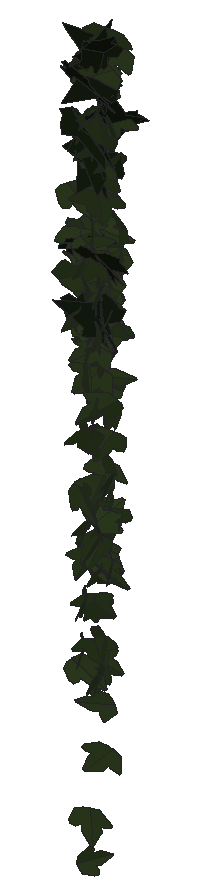
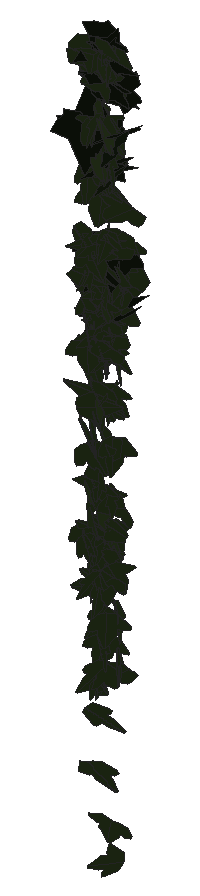
# SketchUp Ruby script. Lengths in inches.
U = 1.inch
M = Sketchup.active_model
def pt(a) = Geom::Point3d.new(a.map { |v| v * U })
def face(e, loops, mat)
  f = e.add_face(loops[0].map { |a| pt(a) })
  loops[1..].each { |l| e.add_face(l.map { |a| pt(a) }).erase! }
  f.material = f.back_material = mat if mat
  f
end
# faces: each face lists its corners as indices into pts; further lists are holes
def faces(e, pts, list, mat = nil) = list.each { |f| face(e, (f[0].is_a?(Array) ? f : [f]).map { |l| l.map { |i| pts[i] } }, mat) }
# xy, xz, yz: faces in a plane at the given z, y or x. An outline is a flat list of corners, or four numbers for a rectangle; further outlines are holes
def ring(l) = l.size == 4 ? [[l[0], l[1]], [l[2], l[1]], [l[2], l[3]], [l[0], l[3]]] : l.each_slice(2).to_a
def flat(e, list, mat, &to3) = list.each { |f| face(e, (f[0].is_a?(Array) ? f : [f]).map { |l| ring(l).map { |u, v| to3.(u, v) } }, mat) }
def xy(e, z, list, mat = nil) = flat(e, list, mat) { |x, y| [x, y, z] }
def xz(e, y, list, mat = nil) = flat(e, list, mat) { |x, z| [x, y, z] }
def yz(e, x, list, mat = nil) = flat(e, list, mat) { |y, z| [x, y, z] }
def lines(e, pts, list) = list.each { |a, b| e.add_line(pt(pts[a]), pt(pts[b])) }
# prism: a flat outline (further loops are holes) pulled along v
def prism(e, loops, v, mat = nil)
  f = face(e, loops, mat); d = Geom::Vector3d.new(v.map { |x| x * U })
  f.pushpull(f.normal.samedirection?(d) ? d.length : -d.length)
end
def box(e, o, s, mat = nil) = prism(e, [[o, [o[0] + s[0], o[1], o[2]], [o[0] + s[0], o[1] + s[1], o[2]], [o[0], o[1] + s[1], o[2]]]], [0, 0, s[2]], mat)
def at(x, y, z, deg = 0) = Geom::Transformation.translation(pt([x, y, z])) * Geom::Transformation.rotation(ORIGIN, Z_AXIS, deg.degrees)
def axes(o, x, y, z) = Geom::Transformation.new([*x, 0, *y, 0, *z, 0, *pt(o).to_a, 1])
def part(name) = M.definitions.add(name)
# library, detail: a bought-in or finely detailed component or shape, given as its bounding box
def library(name, o, s) = part(name).tap { |d| box(d.entities, o, s) }
def detail(e, o, s) = box(e.add_group.entities, o, s)
def put(e, d, t, mat = nil) = e.add_instance(d, t).tap { |i| i.material = mat if mat }
def group(e, t, mat = nil) = e.add_group.tap { |g| g.transformation = t; g.material = mat if mat }.entities
root = M.entities
M.materials.add("1026 AP 7946 SUNNY SIDE UP").color = [254, 231, 186]
M.materials.add("efeu1").color = [18, 25, 13]
M.materials.add("efeu2").color = [43, 57, 29]
c1 = part("ivyleaf_10")
p = [[0,0.5,-0.03],[-0.0625,2.02,-0.43],[-0.19,2.01,-0.46],[-0.54,1.05,-0.29],[-0.52,0.625,-0.18],[-0.83,0.76,-0.28],
  [-1.16,0.64,-0.33],[-1.15,0.33,-0.24],[-0.77,-0.39,0.02],[-0.3,-0.51,0.16],[0.04,-0.48,0.23],[-0.02,2.01,-0.4375],
  [-0.06,2.01,-0.43],[0.04,-0.49,0.23],[0.67,-0.49,0.14],[1.38,0.36,-0.2],[1.375,0.51,-0.24],[0.81,0.65,-0.19],
  [0.62,0.59,-0.15],[0.6,1.09,-0.28],[0.5,1.23,-0.31]]
faces(c1.entities,p,[[0,1,2,3,4,5,6,7,8,9,10],[11,12,0,13,14,15,16,17,18,19,20]],"efeu2")
c2 = part("ivyleaf_9")
p = [[1.54,2.16,1.25],[1.36,2.04,1.19],[-0.21,0.99,0.68],[-0.71,1.11,0.82],[-0.85,0.86,0.67],[-0.8,0.17,0.21],
  [-0.9,-0.01,0.1],[-0.67,-0.16,-0.02],[-0.08,-0.08,-0.05],[-0.03,-0.6,-0.4],[0.65,-0.88,-0.66],[0.83,-0.6,-0.49],
  [1.29,-0.42,-0.43],[1.8125,-0.07,-0.26],[1.21,0.44,0.15]]
faces(c2.entities,p,[[0,1,2,3,4,5,6,7,8,9,10,11,12,13,14]],"efeu1")
put(root,c1,axes([99.72,212.89,265.79],[0.20963,-0.19928,-0.11558],[-0.03459,0.11681,-0.24244],[0.35706,0.12832,0.04437]),"1026 AP 7946 SUNNY SIDE UP")
put(root,c1,axes([99.71,212.82,258.59],[-0.10967,-0.17502,0.09917],[0.0083,-0.10456,-0.19055],[0.31472,-0.05823,0.03958]),"1026 AP 7946 SUNNY SIDE UP")
put(root,c2,axes([99.43,212.72,266.84],[0.31388,-0.09577,0.0641],[0.0745,-0.04749,-0.22245],[0.1779,0.18887,-0.01994]),"1026 AP 7946 SUNNY SIDE UP")
put(root,c1,axes([99.67,212.68,263.39],[-0.21121,0.16245,-0.00844],[-0.00702,-0.01574,-0.21886],[-0.2762,-0.12383,0.01201]),"1026 AP 7946 SUNNY SIDE UP")
put(root,c1,axes([99.6,212.76,263.33],[0.11191,0.12241,0.16363],[0.03891,0.1537,-0.14172],[-0.328,0.06,0.03902]),"1026 AP 7946 SUNNY SIDE UP")
put(root,c1,axes([99.68,212.96,264.36],[-0.06538,-0.14862,-0.12234],[0.05479,0.10765,-0.16282],[0.31147,-0.05013,0.00296]),"1026 AP 7946 SUNNY SIDE UP")
put(root,c1,axes([99.73,212.63,257.06],[0.08073,-0.15207,-0.14427],[-0.02745,0.1397,-0.16307],[0.32298,0.04988,0.0222]),"1026 AP 7946 SUNNY SIDE UP")
put(root,c1,axes([99.78,212.84,263.68],[-0.33809,0.0283,0.04927],[-0.08294,-0.02264,-0.2135],[-0.03787,-0.20307,0.02774]),"1026 AP 7946 SUNNY SIDE UP")
put(root,c1,axes([99.47,212.73,264.79],[0.24956,0.06201,0.14942],[0.22192,0.04688,-0.17005],[-0.1316,0.19665,-0.00341]),"1026 AP 7946 SUNNY SIDE UP")
put(root,c2,axes([99.71,212.68,264.04],[0.18303,0.18713,-0.03013],[-0.01459,-0.03032,-0.23149],[-0.32154,0.10789,-0.00664]),"1026 AP 7946 SUNNY SIDE UP")
put(root,c1,axes([99.73,212.67,257.87],[0.09781,-0.19976,-0.09369],[-0.01295,0.09116,-0.21423],[0.34415,0.0602,0.01857]),"1026 AP 7946 SUNNY SIDE UP")
put(root,c1,axes([99.63,212.85,264.03],[0.2659,0.10364,-0.0658],[0.07127,0.04988,0.2009],[0.19298,-0.16123,0.01646]),"1026 AP 7946 SUNNY SIDE UP")
put(root,c1,axes([99.64,213.17,259.77],[0.03737,-0.07858,0.16785],[0.10325,-0.14589,-0.08889],[0.28089,0.06408,0.01034]),"1026 AP 7946 SUNNY SIDE UP")
put(root,c1,axes([99.65,212.67,264.11],[0.31292,0.10004,-0.01636],[-0.01311,-0.02046,-0.2243],[-0.17164,0.18395,-0.0127]),"1026 AP 7946 SUNNY SIDE UP")
put(root,c1,axes([99.73,212.74,260.71],[-0.13107,-0.19878,-0.05344],[0.03373,0.04603,-0.22178],[0.32081,-0.08605,0.00148]),"1026 AP 7946 SUNNY SIDE UP")
put(root,c1,axes([99.72,212.89,266.15],[0.06156,-0.22169,0.11263],[0.02352,-0.10964,-0.23252],[0.38884,0.04173,-0.00377]),"1026 AP 7946 SUNNY SIDE UP")
put(root,c1,axes([99.48,212.96,259.4],[0.09876,-0.03044,-0.17621],[0.27123,-0.0404,0.06806],[-0.08242,-0.16945,0.01285]),"1026 AP 7946 SUNNY SIDE UP")
put(root,c1,axes([99.78,212.65,262.26],[0.1594,-0.16224,-0.14298],[-0.0652,0.13473,-0.19396],[0.32837,0.10551,0.03089]),"1026 AP 7946 SUNNY SIDE UP")
put(root,c1,axes([99.73,212.71,267.33],[-0.06866,-0.17876,-0.13205],[0.04638,0.11789,-0.19457],[0.3635,-0.04881,-0.00012]),"1026 AP 7946 SUNNY SIDE UP")
put(root,c1,axes([99.8,212.875,261.71],[0.32361,-0.03082,-0.09465],[-0.14681,-0.00688,-0.21354],[0.03981,0.2252,-0.01813]),"1026 AP 7946 SUNNY SIDE UP")
put(root,c1,axes([99.67,212.84,262.54],[0.18413,0.16435,0.02627],[0.00623,0.02437,-0.21019],[-0.2815,0.10804,0.01253]),"1026 AP 7946 SUNNY SIDE UP")
put(root,c1,axes([99.56,213.1,262.54],[0.24621,0.05268,0.11592],[0.17996,0.02223,-0.16434],[-0.0947,0.17921,-0.01094]),"1026 AP 7946 SUNNY SIDE UP")
put(root,c1,axes([99.75,212.8,262.54],[-0.02246,0.05833,-0.18849],[-0.06794,-0.17402,-0.06068],[-0.3087,0.03406,0.02707]),"1026 AP 7946 SUNNY SIDE UP")
put(root,c1,axes([99.75,212.91,257.79],[-0.1902,-0.16488,-0.01098],[0.03829,-0.00588,-0.20935],[0.25687,-0.12121,0.02308]),"1026 AP 7946 SUNNY SIDE UP")
put(root,c1,axes([99.68,213.13,261.35],[-0.01788,-0.03334,-0.20266],[0.02103,-0.18887,0.03232],[-0.32488,-0.01039,0.01325]),"1026 AP 7946 SUNNY SIDE UP")
put(root,c1,axes([99.66,212.75,264.28],[-0.23356,-0.10655,-0.10149],[0.16138,0.02713,-0.18267],[0.17836,-0.16407,0.03238]),"1026 AP 7946 SUNNY SIDE UP")
put(root,c2,axes([99.57,212.98,265.41],[0.12092,-0.22723,0.0407],[0.00483,-0.042,-0.24715],[0.36298,0.07625,-0.01027]),"1026 AP 7946 SUNNY SIDE UP")
put(root,c2,axes([100.01,212.83,267.27],[-0.09329,0.09326,0.20094],[-0.24442,0.12251,-0.10931],[-0.256,-0.15095,0.03114]),"1026 AP 7946 SUNNY SIDE UP")
put(root,c1,axes([99.6875,212.99,263.21],[0.0284,-0.09259,0.17846],[0.1149,-0.15484,-0.1008],[0.30454,0.06706,0.02139]),"1026 AP 7946 SUNNY SIDE UP")
put(root,c2,axes([99.54,212.94,265.9375],[0.20032,-0.20581,0.05097],[0.02835,-0.04835,-0.24944],[0.33207,0.12829,-0.00945]),"1026 AP 7946 SUNNY SIDE UP")
put(root,c1,axes([99.76,212.75,263.6875],[-0.01185,-0.22369,-0.08966],[0.03417,0.08481,-0.22937],[0.37515,-0.01479,0.01806]),"1026 AP 7946 SUNNY SIDE UP")
put(root,c1,axes([99.72,212.8125,261.66],[-0.00619,0.20131,-0.05741],[-0.01279,-0.05635,-0.21616],[-0.35459,-0.00148,0.0088]),"1026 AP 7946 SUNNY SIDE UP")
put(root,c1,axes([99.89,212.61,263.74],[-0.3255,-0.00681,0.08531],[-0.13213,-0.03268,-0.20373],[0.03186,-0.2051,0.02669]),"1026 AP 7946 SUNNY SIDE UP")
put(root,c1,axes([99.68,213.11,265.53],[0.00659,-0.15057,-0.14271],[0.03912,-0.13014,0.15865],[-0.33691,-0.01806,0.01563]),"1026 AP 7946 SUNNY SIDE UP")
put(root,c2,axes([99.61,212.71,262.9375],[0.09797,-0.19248,-0.09],[-0.00231,0.08426,-0.21275],[0.35485,0.05369,0.02347]),"1026 AP 7946 SUNNY SIDE UP")
put(root,c1,axes([99.57,212.54,263.4],[-0.14492,-0.10903,0.21456],[0.2313,0.1486,0.14763],[-0.28944,0.17334,0.01055]),"1026 AP 7946 SUNNY SIDE UP")
put(root,c1,axes([99.8,212.67,259.2],[0.02383,-0.21555,0.01858],[-0.00077,-0.01934,-0.22271],[0.34028,0.01505,-0.00181]),"1026 AP 7946 SUNNY SIDE UP")
put(root,c1,axes([99.8,212.87,265.61],[-0.06047,-0.24411,-0.02461],[0.01587,0.02118,-0.25436],[0.38513,-0.0392,0.00662]),"1026 AP 7946 SUNNY SIDE UP")
put(root,c1,axes([99.875,212.74,262.98],[-0.10937,0.16817,0.09587],[-0.17184,0.04746,-0.17708],[-0.27196,-0.09762,0.07333]),"1026 AP 7946 SUNNY SIDE UP")
put(root,c1,axes([99.76,212.52,262.86],[-0.07598,-0.20488,-0.10742],[0.07368,0.09434,-0.21517],[0.35305,-0.06378,0.02179]),"1026 AP 7946 SUNNY SIDE UP")
put(root,c2,axes([99.61,212.8,266.07],[0.02444,-0.23976,-0.05868],[0.04727,0.05714,-0.24486],[0.3841,0.00822,0.03387]),"1026 AP 7946 SUNNY SIDE UP")
put(root,c1,axes([99.89,212.93,262.44],[-0.18006,0.15618,0.05329],[-0.15985,-0.01198,-0.1822],[-0.22651,-0.1157,0.08622]),"1026 AP 7946 SUNNY SIDE UP")
put(root,c1,axes([99.99,213.08,261.42],[-0.04353,-0.0272,-0.19342],[-0.29214,-0.0566,0.03455],[-0.10237,0.17311,-0.01635]),"1026 AP 7946 SUNNY SIDE UP")
put(root,c1,axes([99.76,213.14,264.26],[0.08996,0.16903,-0.05652],[-0.02932,-0.05222,-0.19037],[-0.3003,0.05573,0.00166]),"1026 AP 7946 SUNNY SIDE UP")
put(root,c1,axes([99.78,212.98,263.4375],[-0.23232,0.15061,-0.01937],[0.00495,-0.02438,-0.21768],[-0.25788,-0.13615,0.01327]),"1026 AP 7946 SUNNY SIDE UP")
put(root,c1,axes([99.87,213.13,264.09],[-0.20772,-0.1347,0.05978],[-0.04893,-0.05144,-0.19507],[0.24383,-0.12508,0.01178]),"1026 AP 7946 SUNNY SIDE UP")
put(root,c1,axes([99.76,212.97,267.33],[0.02181,-0.14797,0.15122],[0.08228,-0.13725,-0.15843],[0.3397,0.04275,0.02867]),"1026 AP 7946 SUNNY SIDE UP")
put(root,c1,axes([99.86,212.8125,262.4],[0.09217,-0.16964,-0.14798],[-0.04597,0.14038,-0.1835],[0.34551,0.06393,0.01507]),"1026 AP 7946 SUNNY SIDE UP")
put(root,c1,axes([99.84,212.9375,258.3],[-0.03912,-0.1684,-0.12235],[0.03346,0.11592,-0.17466],[0.32143,-0.03256,0.00329]),"1026 AP 7946 SUNNY SIDE UP")
put(root,c1,axes([99.86,212.89,258.8],[-0.13209,-0.16377,0.10228],[0.02754,-0.11547,-0.17994],[0.30064,-0.06138,0.06142]),"1026 AP 7946 SUNNY SIDE UP")
put(root,c1,axes([99.87,212.88,259.85],[-0.15504,-0.1755,0.07849],[0.0155,-0.09133,-0.20147],[0.30107,-0.08567,0.05079]),"1026 AP 7946 SUNNY SIDE UP")
put(root,c1,axes([99.85,213.02,266.33],[-0.08253,0.17169,0.10198],[-0.0626,0.08606,-0.18949],[-0.32551,-0.06008,0.01059]),"1026 AP 7946 SUNNY SIDE UP")
put(root,c1,axes([99.88,212.98,260.24],[-0.24772,0.11785,0.02367],[-0.06415,-0.01462,-0.19751],[-0.19269,-0.14665,0.03532]),"1026 AP 7946 SUNNY SIDE UP")
put(root,c1,axes([99.88,213,263.18],[0.28881,0.0163,-0.07335],[-0.1124,-0.02557,-0.18234],[-0.04173,0.1817,-0.01648]),"1026 AP 7946 SUNNY SIDE UP")
put(root,c1,axes([99.6,212.71,259.67],[0.1807,-0.05132,0.20716],[0.29704,-0.0701,-0.12987],[0.13618,0.22101,0.0084]),"1026 AP 7946 SUNNY SIDE UP")
put(root,c1,axes([100,212.82,266.98],[0.26947,-0.02281,-0.15847],[-0.25095,0.00793,-0.17127],[0.03755,0.2167,-0.00735]),"1026 AP 7946 SUNNY SIDE UP")
put(root,c2,axes([99.75,212.97,265.53],[-0.06614,-0.23957,0.02343],[0.00444,-0.02496,-0.25062],[0.37858,-0.04156,0.00703]),"1026 AP 7946 SUNNY SIDE UP")
put(root,c2,axes([99.87,212.95,265.48],[-0.25906,-0.17717,0.02928],[-0.00619,-0.03636,-0.24845],[0.28233,-0.16336,0.02142]),"1026 AP 7946 SUNNY SIDE UP")
put(root,c1,axes([99.86,212.81,258.91],[-0.04471,-0.17727,0.11893],[0.01916,-0.11867,-0.18372],[0.33295,-0.01698,0.02654]),"1026 AP 7946 SUNNY SIDE UP")
put(root,c1,axes([100.03,212.84,256.1],[0.12344,-0.03705,-0.16895],[-0.2661,0.02588,-0.08373],[0.06687,0.17138,-0.02133]),"1026 AP 7946 SUNNY SIDE UP")
put(root,c1,axes([99.68,212.93,258.52],[0.24318,0.08592,0.10846],[0.16285,0.0276,-0.18061],[-0.13741,0.18476,-0.02211]),"1026 AP 7946 SUNNY SIDE UP")
put(root,c1,axes([99.97,212.69,262.26],[0.26685,-0.02622,-0.12433],[-0.19896,-0.00358,-0.16952],[0.03219,0.19521,-0.01704]),"1026 AP 7946 SUNNY SIDE UP")
put(root,c1,axes([99.89,213.01,262.48],[-0.32273,-0.04531,0.00898],[-0.00723,-0.02066,-0.20852],[0.07807,-0.1892,0.0178]),"1026 AP 7946 SUNNY SIDE UP")
put(root,c1,axes([99.88,212.75,259.44],[0.12637,-0.19207,-0.05827],[-0.02416,0.05367,-0.21408],[0.31343,0.08158,0.00699]),"1026 AP 7946 SUNNY SIDE UP")
put(root,c2,axes([100,212.83,266.87],[-0.36149,-0.02607,0.01066],[-0.0128,-0.02267,-0.22884],[0.04582,-0.21199,0.02013]),"1026 AP 7946 SUNNY SIDE UP")
put(root,c1,axes([99.78,212.86,265.47],[0.14483,0.17853,0.01203],[0.01917,0.00447,-0.21158],[-0.30283,0.08567,-0.00764]),"1026 AP 7946 SUNNY SIDE UP")
put(root,c1,axes([99.83,213.0625,262.64],[0.12809,0.15293,-0.06219],[-0.02716,-0.05896,-0.183],[-0.27759,0.07633,-0.01079]),"1026 AP 7946 SUNNY SIDE UP")
put(root,c1,axes([100.13,212.8,265.19],[-0.11635,0.0385,0.20644],[-0.33293,-0.01067,-0.07269],[-0.00455,-0.20389,0.03983]),"1026 AP 7946 SUNNY SIDE UP")
put(root,c1,axes([99.89,212.9,266.36],[0.12772,-0.2384,0.02168],[0.00775,-0.02198,-0.25958],[0.37643,0.08134,-0.00201]),"1026 AP 7946 SUNNY SIDE UP")
put(root,c1,axes([99.94,212.89,263.92],[-0.1327,-0.17221,0.13889],[-0.01884,-0.14166,-0.19358],[0.34433,-0.07412,0.04293]),"1026 AP 7946 SUNNY SIDE UP")
put(root,c2,axes([99.78,212.9375,266.94],[-0.21795,-0.05927,-0.16743],[0.26077,0.03369,-0.14895],[0.10911,-0.19891,0.02156]),"1026 AP 7946 SUNNY SIDE UP")
put(root,c1,axes([100.08,212.89,263.27],[0.11067,0.06474,0.19275],[-0.24796,-0.10462,0.0959],[0.20768,-0.15942,0.01179]),"1026 AP 7946 SUNNY SIDE UP")
put(root,c1,axes([99.96,213.03,259.59],[-0.11479,0.16628,0.02517],[-0.13446,-0.01141,-0.17368],[-0.25081,-0.06998,0.0816]),"1026 AP 7946 SUNNY SIDE UP")
put(root,c1,axes([100.0625,213.13,263.71],[0.13024,0.01188,-0.17488],[-0.26668,-0.04625,-0.08317],[-0.07951,0.17459,-0.00751]),"1026 AP 7946 SUNNY SIDE UP")
put(root,c1,axes([99.84,212.79,263.52],[-0.14284,0.16137,-0.07177],[0.03971,-0.06568,-0.19551],[-0.29535,-0.08687,0.00842]),"1026 AP 7946 SUNNY SIDE UP")
put(root,c1,axes([99.89,212.89,259.07],[-0.03546,-0.16261,-0.13275],[0.05824,0.12344,-0.16764],[0.32008,-0.04048,0.0158]),"1026 AP 7946 SUNNY SIDE UP")
put(root,c1,axes([99.72,212.5625,256.78],[0.15843,0.11621,0.14586],[0.17212,0.09043,-0.15691],[-0.22993,0.14777,-0.01696]),"1026 AP 7946 SUNNY SIDE UP")
put(root,c1,axes([99.94,212.8,262.29],[0.2969,0.02888,0.06325],[-0.10384,0.01273,0.18857],[0.03941,-0.18405,0.02032]),"1026 AP 7946 SUNNY SIDE UP")
put(root,c1,axes([99.81,213.04,258.55],[-0.08595,-0.16722,-0.10388],[0.16677,0.06146,-0.16544],[0.25689,-0.09585,0.07265]),"1026 AP 7946 SUNNY SIDE UP")
put(root,c1,axes([99.96,212.89,263.9375],[-0.10493,-0.21002,0.08316],[-0.01326,-0.08305,-0.2269],[0.35422,-0.06532,0.01614]),"1026 AP 7946 SUNNY SIDE UP")
put(root,c1,axes([99.88,213.01,261.69],[0.15436,-0.15153,0.06225],[0.04208,-0.05519,-0.18982],[0.27352,0.09401,-0.00593]),"1026 AP 7946 SUNNY SIDE UP")
put(root,c1,axes([99.76,212.76,260.59],[-0.21246,0.07996,0.16891],[0.24435,-0.05535,0.15985],[0.14901,0.20477,-0.02128]),"1026 AP 7946 SUNNY SIDE UP")
put(root,c1,axes([99.97,212.65,259.3],[-0.15852,0.12312,0.09725],[-0.10792,0.06351,-0.16416],[-0.23448,-0.11247,0.00981]),"1026 AP 7946 SUNNY SIDE UP")
put(root,c1,axes([99.99,212.97,260.63],[-0.23357,-0.12632,0.09428],[-0.04817,-0.10123,-0.19426],[0.24116,-0.14256,0.0525]),"1026 AP 7946 SUNNY SIDE UP")
put(root,c1,axes([99.74,212.95,262.89],[0.26415,0.06139,0.09711],[0.15386,0.01384,-0.17786],[-0.10238,0.17918,-0.01673]),"1026 AP 7946 SUNNY SIDE UP")
put(root,c1,axes([99.96,212.92,266.14],[-0.10555,-0.23942,0.02321],[0.00017,-0.02484,-0.25621],[0.37834,-0.06678,0.00659]),"1026 AP 7946 SUNNY SIDE UP")
put(root,c1,axes([100.06,212.5,261.17],[0.04787,-0.00976,0.22041],[-0.25706,0.14017,0.03125],[-0.23766,-0.15358,0.01058]),"1026 AP 7946 SUNNY SIDE UP")
put(root,c1,axes([99.96,213.12,262.45],[-0.28554,-0.06488,0.01595],[-0.01364,-0.02269,-0.19234],[0.1125,-0.16741,0.01716]),"1026 AP 7946 SUNNY SIDE UP")
put(root,c1,axes([99.95,212.97,267.56],[-0.3621,-0.00606,0.00491],[-0.00679,-0.0226,-0.2275],[0.01106,-0.21216,0.0211]),"1026 AP 7946 SUNNY SIDE UP")
put(root,c1,axes([99.99,212.89,255.21],[0.28011,-0.00813,-0.09878],[-0.15114,-0.00747,-0.18344],[0.00567,0.20215,-0.00956]),"1026 AP 7946 SUNNY SIDE UP")
put(root,c1,axes([99.86,213.07,262.74],[0.0668,0.17336,0.00429],[0.00772,0.00076,-0.19025],[-0.2942,0.03938,-0.00402]),"1026 AP 7946 SUNNY SIDE UP")
put(root,c1,axes([99.93,213.02,261.1],[0.15153,-0.18608,-0.06393],[-0.00281,0.06715,-0.21353],[0.3079,0.09219,0.02951]),"1026 AP 7946 SUNNY SIDE UP")
put(root,c1,axes([99.96,213.14,259.15],[-0.06244,-0.16879,0.04353],[0.00657,-0.04459,-0.18505],[0.29554,-0.03467,0.01331]),"1026 AP 7946 SUNNY SIDE UP")
put(root,c1,axes([99.77,212.79,264.24],[0.05197,-0.0281,0.2279],[0.23721,-0.16114,-0.04646],[0.27756,0.14298,-0.00297]),"1026 AP 7946 SUNNY SIDE UP")
put(root,c1,axes([100.03,212.79,262.63],[0.12127,0.01111,0.19576],[-0.18808,0.15875,0.03826],[-0.24735,-0.11526,0.06689]),"1026 AP 7946 SUNNY SIDE UP")
put(root,c2,axes([100.14,212.7,262.77],[-0.05814,0.01898,0.24739],[-0.34913,-0.09662,-0.02793],[0.14644,-0.22281,0.03162]),"1026 AP 7946 SUNNY SIDE UP")
put(root,c1,axes([99.9,212.78,257.8],[-0.09555,-0.14677,-0.14186],[0.1141,0.11726,-0.16204],[0.2942,-0.09315,0.01677]),"1026 AP 7946 SUNNY SIDE UP")
put(root,c1,axes([99.89,212.52,253.46],[-0.01342,-0.0236,0.2097],[0.02588,0.20313,0.02614],[-0.32138,0.01734,-0.00665]),"1026 AP 7946 SUNNY SIDE UP")
put(root,c1,axes([99.84,212.66,254.1875],[0.30971,0.01434,0.05788],[0.08954,-0.01196,-0.20289],[-0.01648,0.20445,-0.01472]),"1026 AP 7946 SUNNY SIDE UP")
put(root,c1,axes([99.82,212.64,264.05],[0.20373,0.11893,0.13439],[0.09855,0.11426,-0.17591],[-0.27447,0.1293,0.03658]),"1026 AP 7946 SUNNY SIDE UP")
put(root,c1,axes([99.96,212.9,262.27],[-0.00589,0.02672,0.19943],[0.03488,-0.18479,0.02626],[0.31696,0.02083,0.00081]),"1026 AP 7946 SUNNY SIDE UP")
put(root,c1,axes([99.97,212.76,263.28],[0.12686,-0.21658,-0.05227],[0.00232,0.05319,-0.23694],[0.34933,0.0783,0.02056]),"1026 AP 7946 SUNNY SIDE UP")
put(root,c1,axes([100,212.57,262.66],[0.25086,-0.13998,-0.11083],[-0.05904,0.11374,-0.21072],[0.27047,0.15466,0.05679]),"1026 AP 7946 SUNNY SIDE UP")
put(root,c1,axes([99.99,212.9,266.1875],[-0.21997,0.20168,0.04268],[-0.05855,0.02307,-0.2521],[-0.31804,-0.14374,0.01689]),"1026 AP 7946 SUNNY SIDE UP")
put(root,c1,axes([99.92,212.97,260.08],[0.3165,0.00632,-0.00243],[-0.00251,-0.0251,-0.19827],[-0.01117,0.18477,-0.02422]),"1026 AP 7946 SUNNY SIDE UP")
put(root,c1,axes([99.99,212.71,264.87],[-0.33176,-0.11899,-0.01717],[0.03516,-0.00719,-0.24895],[0.18548,-0.21147,0.01649]),"1026 AP 7946 SUNNY SIDE UP")
put(root,c2,axes([99.95,212.62,267.22],[-0.06822,-0.05893,0.23172],[0.22522,0.17203,0.07864],[-0.30861,0.13857,0.00617]),"1026 AP 7946 SUNNY SIDE UP")
put(root,c1,axes([99.77,212.87,263.61],[0.26304,-0.05081,-0.13965],[0.21833,-0.02264,0.17357],[-0.09115,-0.20085,0.01274]),"1026 AP 7946 SUNNY SIDE UP")
put(root,c2,axes([100.05,212.56,263.96],[0.22762,0.11494,-0.13065],[-0.1664,-0.07538,-0.19004],[-0.23315,0.16601,0.00808]),"1026 AP 7946 SUNNY SIDE UP")
put(root,c1,axes([99.93,213.13,263.77],[-0.17976,0.12307,-0.08968],[0.06045,-0.08087,-0.17323],[-0.24698,-0.10937,0.02288]),"1026 AP 7946 SUNNY SIDE UP")
put(root,c1,axes([99.9,212.8,256.85],[-0.12246,-0.13996,-0.16581],[0.17558,0.11826,-0.16171],[0.28465,-0.13316,0.02841]),"1026 AP 7946 SUNNY SIDE UP")
put(root,c1,axes([99.77,212.88,265.23],[0.20988,0.0136,0.16431],[0.2612,-0.0151,-0.13163],[0.00555,0.19637,-0.01873]),"1026 AP 7946 SUNNY SIDE UP")
put(root,c1,axes([100.02,212.89,262.06],[-0.02934,-0.18167,0.01511],[0.00052,-0.01658,-0.19559],[0.30966,-0.01719,0.00176]),"1026 AP 7946 SUNNY SIDE UP")
put(root,c1,axes([100.02,212.82,256.625],[-0.02937,0.14108,-0.11828],[-0.08557,-0.11213,-0.14402],[-0.29392,0.01855,0.05375]),"1026 AP 7946 SUNNY SIDE UP")
put(root,c1,axes([100.04,212.6875,265.9],[-0.35683,0.04031,-0.00285],[-0.00106,0.01361,0.22889],[0.06864,0.20978,-0.01125]),"1026 AP 7946 SUNNY SIDE UP")
put(root,c1,axes([99.82,212.92,258.4],[-0.19135,0.01399,-0.17319],[0.25741,-0.04066,-0.12574],[-0.06456,-0.20358,0.01197]),"1026 AP 7946 SUNNY SIDE UP")
put(root,c1,axes([99.87,212.9375,266.96],[-0.22712,0.03836,-0.15947],[0.17771,-0.12276,-0.13577],[-0.19243,-0.15864,0.06283]),"1026 AP 7946 SUNNY SIDE UP")
put(root,c2,axes([99.9,212.5625,267.4375],[0.18484,0.13592,0.15727],[0.16083,0.11001,-0.18486],[-0.29675,0.14428,-0.00223]),"1026 AP 7946 SUNNY SIDE UP")
put(root,c1,axes([99.73,212.97,261.62],[0.07235,-0.01742,-0.22502],[0.34439,0.00346,0.04729],[-0.00031,-0.22309,0.01699]),"1026 AP 7946 SUNNY SIDE UP")
put(root,c1,axes([99.88,212.84,259.23],[0.21932,0.05236,-0.16148],[0.15841,0.1361,0.13973],[0.20655,-0.15998,0.0643]),"1026 AP 7946 SUNNY SIDE UP")
put(root,c1,axes([100.13,212.97,267.32],[0.29654,-0.01862,-0.12862],[-0.20441,-0.00079,-0.1877],[0.0253,0.21187,-0.00902]),"1026 AP 7946 SUNNY SIDE UP")
put(root,c1,axes([100.05,212.69,257.29],[0.20612,-0.15229,-0.0914],[-0.04265,0.09077,-0.20323],[0.27314,0.12909,0.03725]),"1026 AP 7946 SUNNY SIDE UP")
put(root,c1,axes([99.97,213.19,263.75],[-0.05585,0.1327,-0.11994],[0.01511,-0.11434,-0.14714],[-0.29633,-0.03084,0.0151]),"1026 AP 7946 SUNNY SIDE UP")
put(root,c1,axes([100.04,212.76,262.64],[0.0544,-0.20197,-0.11545],[0.00463,0.11254,-0.2095],[0.36228,0.02889,0.02001]),"1026 AP 7946 SUNNY SIDE UP")
put(root,c1,axes([99.82,212.91,264.2],[-0.06959,-0.07537,-0.18433],[0.28593,0.06134,-0.07123],[0.13808,-0.165,0.05461]),"1026 AP 7946 SUNNY SIDE UP")
put(root,c2,axes([100.09,212.85,262.46],[0.06978,-0.17682,0.11412],[-0.01378,0.10957,0.19526],[-0.35225,-0.03931,0.01497]),"1026 AP 7946 SUNNY SIDE UP")
put(root,c1,axes([100.15,212.74,261.35],[-0.11883,-0.12591,0.19747],[-0.11641,-0.17842,-0.15129],[0.3423,-0.10439,0.0171]),"1026 AP 7946 SUNNY SIDE UP")
put(root,c1,axes([100,212.62,257.23],[-0.23232,-0.13557,-0.05109],[0.08551,0.0139,-0.20431],[0.22746,-0.14369,0.02462]),"1026 AP 7946 SUNNY SIDE UP")
put(root,c1,axes([99.97,213.12,259.2],[0.19827,-0.13426,0.02331],[0.05562,-0.00242,-0.18896],[0.2246,0.11912,0.02622]),"1026 AP 7946 SUNNY SIDE UP")
put(root,c1,axes([100.05,213.06,259.29],[-0.1774,-0.14022,0.02507],[0.01236,-0.03652,-0.18543],[0.24155,-0.10111,0.0279]),"1026 AP 7946 SUNNY SIDE UP")
put(root,c1,axes([100.05,212.75,262.93],[-0.07352,0.18883,0.05571],[-0.08071,0.03905,-0.20315],[-0.32142,-0.05299,0.03827]),"1026 AP 7946 SUNNY SIDE UP")
put(root,c1,axes([99.98,212.89,266.17],[0.30711,0.15508,0.00606],[-0.04271,0.04209,-0.25149],[-0.2402,0.19079,0.05246]),"1026 AP 7946 SUNNY SIDE UP")
put(root,c1,axes([99.89,212.65,262.68],[0.1648,0.15349,0.09781],[0.09992,0.06827,-0.19306],[-0.28445,0.11291,-0.01115]),"1026 AP 7946 SUNNY SIDE UP")
put(root,c1,axes([100.07,213.04,261.05],[0.15528,-0.14878,-0.05396],[-0.05051,0.03857,-0.18636],[0.26077,0.09606,-0.00397]),"1026 AP 7946 SUNNY SIDE UP")
put(root,c1,axes([99.94,212.95,261.31],[0.09903,-0.11767,0.13841],[0.13631,-0.10483,-0.14075],[0.26578,0.09761,0.02061]),"1026 AP 7946 SUNNY SIDE UP")
put(root,c2,axes([99.99,212.63,263.87],[0.32319,-0.01256,-0.13102],[-0.20159,0.03902,-0.20179],[0.05351,0.22285,0.03116]),"1026 AP 7946 SUNNY SIDE UP")
put(root,c1,axes([100.05,212.93,265.375],[-0.09605,-0.22713,-0.07011],[0.04626,0.06114,-0.24163],[0.36937,-0.06672,0.01203]),"1026 AP 7946 SUNNY SIDE UP")
put(root,c1,axes([100.0625,212.89,258.5],[0.12041,-0.16749,-0.10745],[-0.00986,0.10877,-0.18574],[0.30931,0.06867,0.03591]),"1026 AP 7946 SUNNY SIDE UP")
put(root,c1,axes([100.06,212.6,256.7],[-0.00979,-0.16202,-0.14244],[0.02181,0.1368,-0.1661],[0.33326,-0.01371,0.00668]),"1026 AP 7946 SUNNY SIDE UP")
put(root,c1,axes([100.1875,212.99,264.28],[0.11183,-0.04364,-0.19338],[-0.17649,0.14947,-0.07742],[0.26033,0.12009,0.03058]),"1026 AP 7946 SUNNY SIDE UP")
put(root,c1,axes([100.07,212.91,259.99],[0.0832,-0.21174,0.00966],[0.00024,-0.01087,-0.22489],[0.33335,0.05285,-0.00225]),"1026 AP 7946 SUNNY SIDE UP")
put(root,c2,axes([100.08,212.95,266.15],[0.15367,0.22389,-0.04917],[-0.01224,-0.05,-0.25163],[-0.36018,0.09722,-0.01243]),"1026 AP 7946 SUNNY SIDE UP")
put(root,c1,axes([100.06,212.98,262.875],[0.1009,-0.21578,-0.04231],[0.01563,0.04433,-0.23057],[0.34468,0.06116,0.02284]),"1026 AP 7946 SUNNY SIDE UP")
put(root,c1,axes([100.03,212.85,263.12],[-0.14668,-0.21625,-0.01292],[0.09143,-0.01315,-0.23509],[0.328,-0.09304,0.05975]),"1026 AP 7946 SUNNY SIDE UP")
put(root,c2,axes([99.97,212.91,266.03],[0.30722,0.0997,0.12006],[-0.17681,-0.03389,0.22497],[0.163,-0.22467,0.01774]),"1026 AP 7946 SUNNY SIDE UP")
